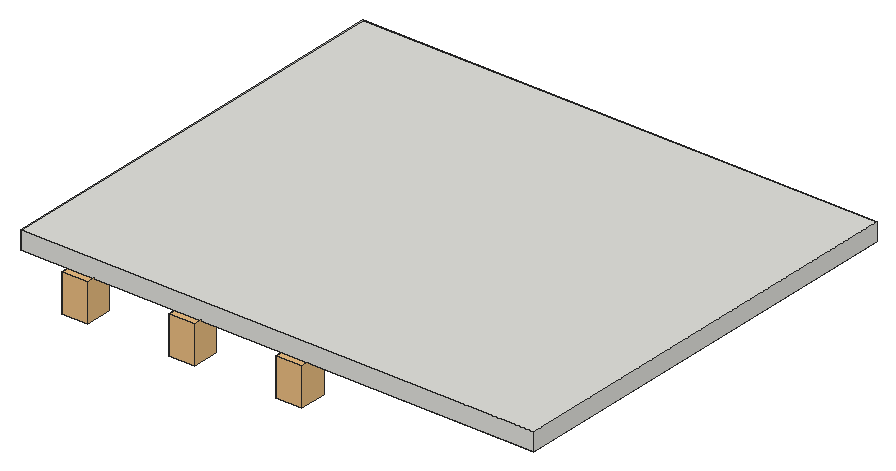
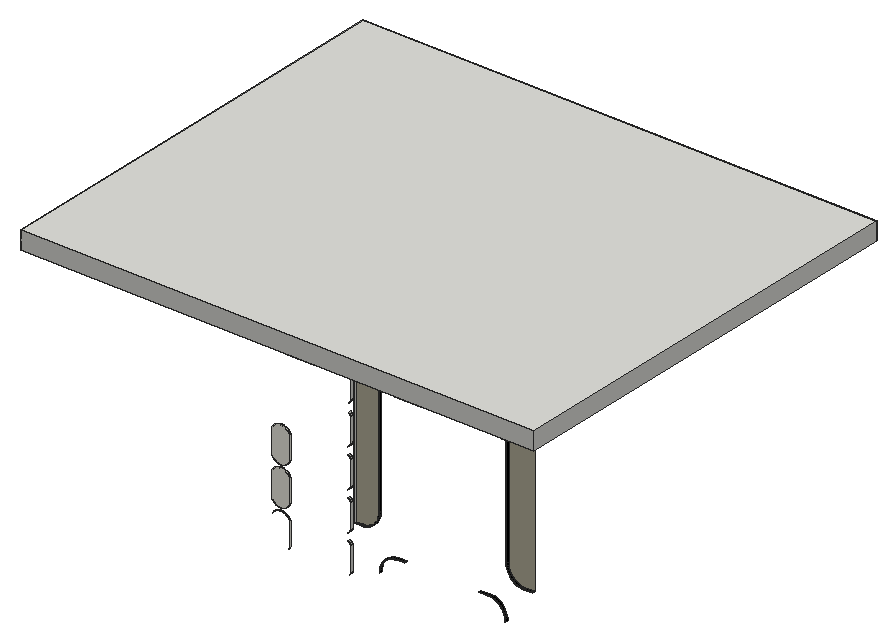
# SketchUp Ruby script. Lengths in inches.
U = 1.inch
M = Sketchup.active_model
def pt(a) = Geom::Point3d.new(a.map { |v| v * U })
def face(e, loops, mat)
  f = e.add_face(loops[0].map { |a| pt(a) })
  loops[1..].each { |l| e.add_face(l.map { |a| pt(a) }).erase! }
  f.material = f.back_material = mat if mat
  f
end
# faces: each face lists its corners as indices into pts; further lists are holes
def faces(e, pts, list, mat = nil) = list.each { |f| face(e, (f[0].is_a?(Array) ? f : [f]).map { |l| l.map { |i| pts[i] } }, mat) }
# xy, xz, yz: faces in a plane at the given z, y or x. An outline is a flat list of corners, or four numbers for a rectangle; further outlines are holes
def ring(l) = l.size == 4 ? [[l[0], l[1]], [l[2], l[1]], [l[2], l[3]], [l[0], l[3]]] : l.each_slice(2).to_a
def flat(e, list, mat, &to3) = list.each { |f| face(e, (f[0].is_a?(Array) ? f : [f]).map { |l| ring(l).map { |u, v| to3.(u, v) } }, mat) }
def xy(e, z, list, mat = nil) = flat(e, list, mat) { |x, y| [x, y, z] }
def xz(e, y, list, mat = nil) = flat(e, list, mat) { |x, z| [x, y, z] }
def yz(e, x, list, mat = nil) = flat(e, list, mat) { |y, z| [x, y, z] }
def lines(e, pts, list) = list.each { |a, b| e.add_line(pt(pts[a]), pt(pts[b])) }
# prism: a flat outline (further loops are holes) pulled along v
def prism(e, loops, v, mat = nil)
  f = face(e, loops, mat); d = Geom::Vector3d.new(v.map { |x| x * U })
  f.pushpull(f.normal.samedirection?(d) ? d.length : -d.length)
end
def box(e, o, s, mat = nil) = prism(e, [[o, [o[0] + s[0], o[1], o[2]], [o[0] + s[0], o[1] + s[1], o[2]], [o[0], o[1] + s[1], o[2]]]], [0, 0, s[2]], mat)
def at(x, y, z, deg = 0) = Geom::Transformation.translation(pt([x, y, z])) * Geom::Transformation.rotation(ORIGIN, Z_AXIS, deg.degrees)
def axes(o, x, y, z) = Geom::Transformation.new([*x, 0, *y, 0, *z, 0, *pt(o).to_a, 1])
def part(name) = M.definitions.add(name)
# library, detail: a bought-in or finely detailed component or shape, given as its bounding box
def library(name, o, s) = part(name).tap { |d| box(d.entities, o, s) }
def detail(e, o, s) = box(e.add_group.entities, o, s)
def put(e, d, t, mat = nil) = e.add_instance(d, t).tap { |i| i.material = mat if mat }
def group(e, t, mat = nil) = e.add_group.tap { |g| g.transformation = t; g.material = mat if mat }.entities
root = M.entities
M.materials.add("Tafisa-Gardenia-or-Gardenia-PM775-4K").color = [246, 245, 235]
M.materials.add("Uniboard-L19-Putty-4K").color = [187, 181, 160]
M.materials.add("[Color M09]").color = [0, 0, 0]
c1 = library("Group\#8",[0,0,0],[8.9,8.9,12.62])
xy(root,61.26,[[19.5,138,22.5,138.71],[47.5,138,50,138.71]],"[Color M09]")
xy(root,61.5,[[19.5,138,22.5,138.71],[47.5,138,50,138.71]],"[Color M09]")
xy(root,67.3125,[[4.5,138,7.5,138.71],[62,138,64.38,138.71]],"[Color M09]")
xy(root,67.55,[[4.5,138,7.5,138.71],[62,138,64.38,138.71]],"[Color M09]")
xz(root,138,[[4.5,67.55,7.5,67.55,8.25,67.6,8.99,67.75,9.71,67.99,10.38,68.32,11.01,68.74,11.58,69.24,12.07,69.8,12.49,70.43,12.83,71.11,13.07,71.82,13.21,72.56,13.26,73.3125,13.26,114,4.5,114],[62,67.55,64.38,67.55,64.38,114,56.24,114,56.24,73.3125,56.29,72.56,56.43,71.82,56.67,71.11,57.01,70.43,57.43,69.8,57.92,69.24,58.49,68.74,59.12,68.32,59.79,67.99,60.51,67.75,61.25,67.6]],"Uniboard-L19-Putty-4K")
xz(root,138.25,[[89.53,63,89.85,63.02,90.17,63.0625,90.48,63.14,90.78,63.25,91.07,63.38,91.35,63.55,91.61,63.73,91.84,63.95,92.0625,64.18,92.25,64.4375,92.42,64.71,92.5625,65,92.5625,73,92.42,73.29,92.25,73.5625,92.0625,73.82,91.84,74.05,91.61,74.27,91.35,74.45,91.07,74.62,90.78,74.75,90.48,74.86,90.17,74.9375,89.85,74.98,89.53,75,89.21,74.98,89.02,74.96,88.89,74.9375,88.58,74.86,88.28,74.75,87.99,74.62,87.72,74.45,87.46,74.27,87.22,74.05,87,73.82,86.81,73.5625,86.64,73.29,86.5,73,86.5,65,86.64,64.71,86.81,64.4375,87,64.18,87.22,63.95,87.46,63.73,87.72,63.55,87.99,63.38,88.28,63.25,88.58,63.14,88.89,63.0625,89.02,63.04,89.21,63.02],[89.53,76,89.85,76.02,90.17,76.0625,90.48,76.14,90.78,76.25,91.07,76.38,91.35,76.55,91.61,76.73,91.84,76.95,92.0625,77.18,92.25,77.4375,92.42,77.71,92.5625,78,92.5625,86,92.42,86.29,92.25,86.5625,92.0625,86.82,91.84,87.05,91.61,87.27,91.35,87.45,91.07,87.62,90.78,87.75,90.48,87.86,90.17,87.9375,89.85,87.98,89.53,88,89.21,87.98,88.89,87.9375,88.58,87.86,88.28,87.75,87.99,87.62,87.72,87.45,87.46,87.27,87.22,87.05,87,86.82,86.81,86.5625,86.64,86.29,86.5,86,86.5,78,86.64,77.71,86.81,77.4375,87,77.18,87.22,76.95,87.46,76.73,87.72,76.55,87.99,76.38,88.28,76.25,88.58,76.14,88.89,76.0625,89.02,76.04,89.21,76.02]],"Tafisa-Gardenia-or-Gardenia-PM775-4K")
yz(root,13.26,[[138,73.3125,138.71,114]],"[Color M09]")
yz(root,13.5,[[138,73.3125,138.71,114]],"[Color M09]")
yz(root,56,[[138,73.3125,138.71,114]],"[Color M09]")
yz(root,56.24,[[138,73.3125,138.71,114]],"[Color M09]")
yz(root,64.38,[[138,67.55,138.71,114]])
yz(root,64.5,[[138,67.3125,138.71,67.55],[138,67.55,138.71,114]])
yz(root,65.5,[[138,52,138.79,60],[138,65,138.79,73],[138,78,138.79,86],[138,91,138.79,99],[138,104,138.79,112]])
yz(root,86.5,[[138,52,138.25,60],[138,65,138.25,73],[138,78,138.25,86]],"Tafisa-Gardenia-or-Gardenia-PM775-4K")
p = [[65.8,138.79,51.44],[65.64,138.79,51.71],[65.64,138,51.71],[65.8,138,51.44],[86.64,138,51.71],[86.81,138,51.4375],
  [86.81,138.25,51.4375],[86.64,138.25,51.71],[65.5,138.79,52],[65.5,138,52],[86.5,138,52],[86.5,138.25,52],
  [13.55,138,56.28],[13.5,138,55.5],[13.5,138.71,55.5],[13.55,138.71,56.28],[13.74,138,55.5],[13.79,138,56.25],
  [13.79,138.71,56.25],[13.74,138.71,55.5],[55.71,138,56.25],[55.76,138,55.5],[55.76,138.71,55.5],[55.71,138.71,56.25],
  [56,138,55.5],[55.95,138,56.28],[55.95,138.71,56.28],[56,138.71,55.5],[13.7,138,57.05],[13.7,138.71,57.05],
  [13.93,138,56.99],[13.93,138.71,56.99],[55.57,138,56.99],[55.57,138.71,56.99],[55.8,138,57.05],[55.8,138.71,57.05],
  [14.17,138,57.71],[14.17,138.71,57.71],[55.33,138,57.71],[55.33,138.71,57.71],[13.96,138,57.8],[13.96,138.71,57.8],
  [55.54,138,57.8],[55.54,138.71,57.8],[14.51,138,58.38],[14.51,138.71,58.38],[54.99,138,58.38],[54.99,138.71,58.38],
  [14.3,138,58.5],[14.3,138.71,58.5],[55.2,138,58.5],[55.2,138.71,58.5],[14.93,138,59.01],[14.93,138.71,59.01],
  [54.57,138,59.01],[54.57,138.71,59.01],[14.74,138,59.15],[14.74,138.71,59.15],[54.76,138,59.15],[54.76,138.71,59.15],
  [15.42,138,59.58],[15.42,138.71,59.58],[54.08,138,59.58],[54.08,138.71,59.58],[15.26,138,59.74],[15.26,138.71,59.74],
  [54.24,138,59.74],[54.24,138.71,59.74],[15.99,138,60.07],[15.99,138.71,60.07],[53.51,138,60.07],[53.51,138.71,60.07],
  [15.85,138,60.26],[15.85,138.71,60.26],[53.65,138,60.26],[53.65,138.71,60.26],[65.5,138.79,60],[65.64,138.79,60.29],
  [65.64,138,60.29],[65.5,138,60],[86.64,138,60.29],[86.5,138,60],[86.5,138.25,60],[86.64,138.25,60.29],
  [16.62,138,60.49],[16.62,138.71,60.49],[52.88,138,60.49],[52.88,138.71,60.49],[16.5,138,60.7],[16.5,138.71,60.7],
  [53,138,60.7],[53,138.71,60.7],[65.8,138.79,60.56],[65.8,138,60.56],[86.81,138,60.5625],[86.81,138.25,60.5625],
  [17.29,138,60.83],[17.29,138.71,60.83],[52.21,138,60.83],[52.21,138.71,60.83],[65.99,138.79,60.82],[65.99,138,60.82],
  [87,138,60.82],[87,138.25,60.82],[92.25,138,60.5625],[92.0625,138,60.82],[92.0625,138.25,60.82],[92.25,138.25,60.5625],
  [17.2,138,61.04],[17.2,138.71,61.04],[52.3,138,61.04],[52.3,138.71,61.04],[18.01,138,61.07],[18.01,138.71,61.07],
  [51.49,138,61.07],[51.49,138.71,61.07],[66.21,138.79,61.05],[66.21,138,61.05],[87.22,138,61.05],[87.22,138.25,61.05],
  [91.84,138,61.05],[91.84,138.25,61.05],[17.95,138,61.3],[17.95,138.71,61.3],[51.55,138,61.3],[51.55,138.71,61.3],
  [18.75,138,61.21],[18.75,138.71,61.21],[50.75,138,61.21],[50.75,138.71,61.21],[66.44,138.79,61.26],[66.44,138,61.26],
  [87.46,138,61.27],[87.46,138.25,61.27],[91.61,138,61.27],[91.61,138.25,61.27],[19.5,138,61.26],[19.5,138.71,61.26],
  [50,138,61.26],[50,138.71,61.26],[18.72,138,61.45],[18.72,138.71,61.45],[50.78,138,61.45],[50.78,138.71,61.45],
  [87.72,138,61.45],[87.72,138.25,61.45],[91.35,138,61.45],[91.35,138.25,61.45],[19.5,138,61.5],[19.5,138.71,61.5],
  [50,138,61.5],[50,138.71,61.5],[87.99,138,61.62],[87.99,138.25,61.62],[91.07,138,61.62],[91.07,138.25,61.62],
  [88.28,138,61.75],[88.28,138.25,61.75],[90.78,138,61.75],[90.78,138.25,61.75],[88.58,138,61.86],[88.58,138.25,61.86],
  [90.48,138,61.86],[90.48,138.25,61.86],[88.89,138,61.9375],[88.89,138.25,61.9375],[89.02,138,61.96],[89.02,138.25,61.96],
  [90.17,138,61.9375],[89.85,138,61.98],[89.85,138.25,61.98],[90.17,138.25,61.9375],[89.21,138,61.98],[89.21,138.25,61.98],
  [89.53,138,62],[89.53,138.25,62],[88.89,138,63.0625],[89.02,138,63.04],[89.02,138.25,63.04],[88.89,138.25,63.0625],
  [89.21,138,63.02],[89.21,138.25,63.02],[89.53,138,63],[89.53,138.25,63],[89.85,138,63.02],[89.85,138.25,63.02],
  [90.17,138,63.0625],[90.17,138.25,63.0625],[88.28,138,63.25],[88.58,138,63.14],[88.58,138.25,63.14],[88.28,138.25,63.25],
  [88.78,138,63.09],[88.78,138.25,63.09],[90.48,138,63.14],[90.48,138.25,63.14],[90.78,138,63.25],[90.78,138.25,63.25],
  [87.99,138,63.38],[87.99,138.25,63.38],[91.07,138,63.38],[91.07,138.25,63.38],[87.72,138,63.55],[87.72,138.25,63.55],
  [91.35,138,63.55],[91.35,138.25,63.55],[87.46,138,63.73],[87.46,138.25,63.73],[91.61,138,63.73],[91.61,138.25,63.73],
  [66.44,138.79,63.74],[66.21,138.79,63.95],[66.21,138,63.95],[66.44,138,63.74],[87.22,138,63.95],[87.22,138.25,63.95],
  [91.84,138,63.95],[91.84,138.25,63.95],[65.99,138.79,64.18],[65.99,138,64.18],[87,138,64.18],[87,138.25,64.18],
  [92.0625,138,64.18],[92.0625,138.25,64.18],[65.8,138.79,64.44],[65.8,138,64.44],[86.81,138,64.4375],[86.81,138.25,64.4375],
  [92.25,138,64.4375],[92.25,138.25,64.4375],[65.64,138.79,64.71],[65.64,138,64.71],[86.64,138,64.71],[86.64,138.25,64.71],
  [65.5,138.79,65],[65.5,138,65],[86.5,138,65],[86.5,138.25,65],[7.5,138,67.3125],[8.28,138,67.36],
  [8.28,138.71,67.36],[7.5,138.71,67.3125],[61.22,138,67.36],[62,138,67.3125],[62,138.71,67.3125],[61.22,138.71,67.36],
  [9.05,138,67.52],[9.05,138.71,67.52],[60.45,138,67.52],[60.45,138.71,67.52],[8.25,138,67.6],[7.5,138,67.55],
  [7.5,138.71,67.55],[8.25,138.71,67.6],[9.8,138,67.77],[9.8,138.71,67.77],[59.7,138,67.77],[59.7,138.71,67.77],
  [62,138,67.55],[61.25,138,67.6],[61.25,138.71,67.6],[62,138.71,67.55],[8.99,138,67.75],[8.99,138.71,67.75],
  [60.51,138,67.75],[60.51,138.71,67.75],[9.71,138,67.99],[9.71,138.71,67.99],[59.79,138,67.99],[59.79,138.71,67.99],
  [10.5,138,68.12],[10.5,138.71,68.12],[59,138,68.12],[59,138.71,68.12],[10.38,138,68.32],[10.38,138.71,68.32],
  [59.12,138,68.32],[59.12,138.71,68.32],[11.15,138,68.55],[11.15,138.71,68.55],[58.35,138,68.55],[58.35,138.71,68.55],
  [11.01,138,68.74],[11.01,138.71,68.74],[58.49,138,68.74],[58.49,138.71,68.74],[11.74,138,69.07],[11.74,138.71,69.07],
  [57.76,138,69.07],[57.76,138.71,69.07],[11.58,138,69.24],[11.58,138.71,69.24],[57.92,138,69.24],[57.92,138.71,69.24],
  [12.26,138,69.66],[12.26,138.71,69.66],[57.24,138,69.66],[57.24,138.71,69.66],[12.07,138,69.8],[12.07,138.71,69.8],
  [57.43,138,69.8],[57.43,138.71,69.8],[12.7,138,70.3125],[12.7,138.71,70.3125],[56.8,138,70.3125],[56.8,138.71,70.3125],
  [12.49,138,70.43],[12.49,138.71,70.43],[57.01,138,70.43],[57.01,138.71,70.43],[13.04,138,71.02],[13.04,138.71,71.02],
  [56.46,138,71.02],[56.46,138.71,71.02],[12.83,138,71.11],[12.83,138.71,71.11],[56.67,138,71.11],[56.67,138.71,71.11],
  [13.3,138,71.76],[13.3,138.71,71.76],[56.2,138,71.76],[56.2,138.71,71.76],[13.07,138,71.82],[13.07,138.71,71.82],
  [56.43,138,71.82],[56.43,138.71,71.82],[13.21,138,72.56],[13.21,138.71,72.56],[13.45,138,72.53],[13.45,138.71,72.53],
  [56.05,138,72.53],[56.05,138.71,72.53],[56.29,138,72.56],[56.29,138.71,72.56],[13.5,138,73.3125],[13.5,138.71,73.3125],
  [56,138,73.3125],[56,138.71,73.3125],[13.26,138,73.3125],[13.26,138.71,73.3125],[56.24,138,73.3125],[56.24,138.71,73.3125],
  [65.5,138.79,73],[65.64,138.79,73.29],[65.64,138,73.29],[65.5,138,73],[86.64,138,73.29],[86.5,138,73],
  [86.5,138.25,73],[86.64,138.25,73.29],[65.8,138.79,73.56],[65.8,138,73.56],[86.81,138,73.5625],[86.81,138.25,73.5625],
  [65.99,138.79,73.82],[65.99,138,73.82],[87,138,73.82],[87,138.25,73.82],[66.21,138.79,74.05],[66.21,138,74.05],
  [87.22,138,74.05],[87.22,138.25,74.05],[92.0625,138,73.82],[91.84,138,74.05],[91.84,138.25,74.05],[92.0625,138.25,73.82],
  [66.44,138.79,74.26],[66.44,138,74.26],[87.46,138,74.27],[87.46,138.25,74.27],[91.61,138,74.27],[91.61,138.25,74.27],
  [87.72,138,74.45],[87.72,138.25,74.45],[91.35,138,74.45],[91.35,138.25,74.45],[87.99,138,74.62],[87.99,138.25,74.62],
  [91.07,138,74.62],[91.07,138.25,74.62],[88.28,138,74.75],[88.28,138.25,74.75],[90.78,138,74.75],[90.78,138.25,74.75],
  [88.58,138,74.86],[88.58,138.25,74.86],[90.48,138,74.86],[90.48,138.25,74.86],[88.89,138,74.9375],[88.89,138.25,74.9375],
  [89.02,138,74.96],[89.02,138.25,74.96],[90.17,138,74.9375],[89.85,138,74.98],[89.85,138.25,74.98],[90.17,138.25,74.9375],
  [89.21,138,74.98],[89.21,138.25,74.98],[89.53,138,75],[89.53,138.25,75],[88.89,138,76.0625],[89.02,138,76.04],
  [89.02,138.25,76.04],[88.89,138.25,76.0625],[89.21,138,76.02],[89.21,138.25,76.02],[89.53,138,76],[89.53,138.25,76],
  [89.85,138,76.02],[89.85,138.25,76.02],[90.17,138,76.0625],[90.17,138.25,76.0625],[88.28,138,76.25],[88.58,138,76.14],
  [88.58,138.25,76.14],[88.28,138.25,76.25],[90.48,138,76.14],[90.48,138.25,76.14],[90.78,138,76.25],[90.78,138.25,76.25],
  [87.99,138,76.38],[87.99,138.25,76.38],[91.07,138,76.38],[91.07,138.25,76.38],[87.72,138,76.55],[87.72,138.25,76.55],
  [91.35,138,76.55],[91.35,138.25,76.55],[87.46,138,76.73],[87.46,138.25,76.73],[91.61,138,76.73],[91.61,138.25,76.73],
  [66.44,138.79,76.74],[66.21,138.79,76.95],[66.21,138,76.95],[66.44,138,76.74],[87.22,138,76.95],[87.22,138.25,76.95],
  [91.84,138,76.95],[91.84,138.25,76.95],[65.99,138.79,77.18],[65.99,138,77.18],[87,138,77.18],[87,138.25,77.18],
  [92.0625,138,77.18],[92.0625,138.25,77.18],[65.8,138.79,77.44],[65.8,138,77.44],[86.81,138,77.4375],[86.81,138.25,77.4375],
  [65.64,138.79,77.71],[65.64,138,77.71],[86.64,138,77.71],[86.64,138.25,77.71],[65.5,138.79,78],[65.5,138,78],
  [86.5,138,78],[86.5,138.25,78],[65.5,138.79,86],[65.64,138.79,86.29],[65.64,138,86.29],[65.5,138,86],
  [86.64,138,86.29],[86.5,138,86],[86.5,138.25,86],[86.64,138.25,86.29],[65.8,138.79,86.56],[65.8,138,86.56],
  [86.81,138,86.5625],[86.81,138.25,86.5625],[65.99,138.79,86.82],[65.99,138,86.82],[87,138,86.82],[87,138.25,86.82],
  [66.21,138.79,87.05],[66.21,138,87.05],[87.22,138,87.05],[87.22,138.25,87.05],[92.0625,138,86.82],[91.84,138,87.05],
  [91.84,138.25,87.05],[92.0625,138.25,86.82],[66.44,138.79,87.26],[66.44,138,87.26],[87.46,138,87.27],[87.46,138.25,87.27],
  [91.61,138,87.27],[91.61,138.25,87.27],[87.72,138,87.45],[87.72,138.25,87.45],[91.35,138,87.45],[91.35,138.25,87.45],
  [87.99,138,87.62],[87.99,138.25,87.62],[91.07,138,87.62],[91.07,138.25,87.62],[88.28,138,87.75],[88.28,138.25,87.75],
  [90.78,138,87.75],[90.78,138.25,87.75],[88.58,138,87.86],[88.58,138.25,87.86],[90.48,138,87.86],[90.48,138.25,87.86],
  [88.89,138,87.9375],[88.89,138.25,87.9375],[89.21,138,87.98],[89.21,138.25,87.98],[90.17,138,87.9375],[89.85,138,87.98],
  [89.85,138.25,87.98],[90.17,138.25,87.9375],[89.53,138,88],[89.53,138.25,88],[66.44,138.79,89.74],[66.21,138.79,89.95],
  [66.21,138,89.95],[66.44,138,89.74],[65.99,138.79,90.18],[65.99,138,90.18],[65.8,138.79,90.44],[65.8,138,90.44],
  [65.64,138.79,90.71],[65.64,138,90.71],[65.5,138.79,91],[65.5,138,91],[65.5,138.79,99],[65.64,138.79,99.29],
  [65.64,138,99.29],[65.5,138,99],[65.8,138.79,99.56],[65.8,138,99.56],[65.99,138.79,99.82],[65.99,138,99.82],
  [66.21,138.79,100.05],[66.21,138,100.05],[66.21,138.79,102.95],[65.99,138.79,103.18],[65.99,138,103.18],[66.21,138,102.95],
  [65.8,138.79,103.44],[65.8,138,103.44],[65.64,138.79,103.71],[65.64,138,103.71],[65.5,138.79,104],[65.5,138,104],
  [65.5,138.79,112],[65.64,138.79,112.29],[65.64,138,112.29],[65.5,138,112],[65.8,138.79,112.56],[65.8,138,112.56],
  [65.99,138.79,112.82],[65.99,138,112.82],[66.21,138.79,113.05],[66.21,138,113.05]]
faces(root,p,[[0,1,2,3],[1,8,9,2],[76,77,78,79],[77,92,93,78],[92,100,101,93],[100,116,117,101],[116,130,131,117],[210,211,212,213],
  [211,218,219,212],[218,224,225,219],[224,230,231,225],[230,234,235,231],[342,343,344,345],[343,350,351,344],[350,354,355,351],[354,358,359,355],
  [358,366,367,359],[432,433,434,435],[433,440,441,434],[440,446,447,441],[446,450,451,447],[450,454,455,451],[458,459,460,461],[459,466,467,460],
  [466,470,471,467],[470,474,475,471],[474,482,483,475],[514,515,516,517],[515,518,519,516],[518,520,521,519],[520,522,523,521],[522,524,525,523],
  [526,527,528,529],[527,530,531,528],[530,532,533,531],[532,534,535,533],[536,537,538,539],[537,540,541,538],[540,542,543,541],[542,544,545,543],
  [546,547,548,549],[547,550,551,548],[550,552,553,551],[552,554,555,553]])
faces(root,p,[[4,5,6,7],[10,4,7,11],[80,81,82,83],[94,80,83,95],[102,94,95,103],[104,105,106,107],[118,102,103,119],[105,120,121,106],
  [132,118,119,133],[120,134,135,121],[144,132,133,145],[134,146,147,135],[152,144,145,153],[146,154,155,147],[156,152,153,157],[154,158,159,155],
  [160,156,157,161],[158,162,163,159],[164,160,161,165],[166,164,165,167],[168,169,170,171],[162,168,171,163],[172,166,167,173],[174,172,173,175],
  [169,174,175,170],[176,177,178,179],[177,180,181,178],[180,182,183,181],[182,184,185,183],[184,186,187,185],[188,189,190,191],[189,192,193,190],
  [192,176,179,193],[186,194,195,187],[194,196,197,195],[198,188,191,199],[196,200,201,197],[202,198,199,203],[200,204,205,201],[206,202,203,207],
  [204,208,209,205],[214,206,207,215],[208,216,217,209],[220,214,215,221],[216,222,223,217],[226,220,221,227],[222,228,229,223],[232,226,227,233],
  [236,232,233,237],[346,347,348,349],[352,346,349,353],[356,352,353,357],[360,356,357,361],[362,363,364,365],[368,360,361,369],[363,370,371,364],
  [372,368,369,373],[370,374,375,371],[376,372,373,377],[374,378,379,375],[380,376,377,381],[378,382,383,379],[384,380,381,385],[382,386,387,383],
  [388,384,385,389],[390,388,389,391],[392,393,394,395],[386,392,395,387],[396,390,391,397],[398,396,397,399],[393,398,399,394],[400,401,402,403],
  [401,404,405,402],[404,406,407,405],[406,408,409,407],[408,410,411,409],[412,413,414,415],[413,400,403,414],[410,416,417,411],[416,418,419,417],
  [420,412,415,421],[418,422,423,419],[424,420,421,425],[422,426,427,423],[428,424,425,429],[426,430,431,427],[436,428,429,437],[430,438,439,431],
  [442,436,437,443],[438,444,445,439],[448,442,443,449],[452,448,449,453],[456,452,453,457],[462,463,464,465],[468,462,465,469],[472,468,469,473],
  [476,472,473,477],[478,479,480,481],[484,476,477,485],[479,486,487,480],[488,484,485,489],[486,490,491,487],[492,488,489,493],[490,494,495,491],
  [496,492,493,497],[494,498,499,495],[500,496,497,501],[498,502,503,499],[504,500,501,505],[506,504,505,507],[508,509,510,511],[502,508,511,503],
  [512,506,507,513],[509,512,513,510]],"Tafisa-Gardenia-or-Gardenia-PM775-4K")
faces(root,p,[[12,13,14,15],[16,17,18,19],[20,21,22,23],[24,25,26,27],[28,12,15,29],[17,30,31,18],[32,20,23,33],[25,34,35,26],
  [30,36,37,31],[38,32,33,39],[40,28,29,41],[34,42,43,35],[36,44,45,37],[46,38,39,47],[48,40,41,49],[42,50,51,43],
  [44,52,53,45],[54,46,47,55],[56,48,49,57],[50,58,59,51],[52,60,61,53],[62,54,55,63],[64,56,57,65],[58,66,67,59],
  [60,68,69,61],[70,62,63,71],[72,64,65,73],[66,74,75,67],[68,84,85,69],[86,70,71,87],[88,72,73,89],[74,90,91,75],
  [84,96,97,85],[98,86,87,99],[108,88,89,109],[90,110,111,91],[96,112,113,97],[114,98,99,115],[122,108,109,123],[110,124,125,111],
  [112,126,127,113],[128,114,115,129],[126,136,137,127],[138,128,129,139],[140,122,123,141],[124,142,143,125],[148,140,141,149],[142,150,151,143],
  [238,239,240,241],[242,243,244,245],[239,246,247,240],[248,242,245,249],[250,251,252,253],[246,254,255,247],[256,248,249,257],[258,259,260,261],
  [262,250,253,263],[259,264,265,260],[266,262,263,267],[264,268,269,265],[254,270,271,255],[272,256,257,273],[274,266,267,275],[268,276,277,269],
  [270,278,279,271],[280,272,273,281],[282,274,275,283],[276,284,285,277],[278,286,287,279],[288,280,281,289],[290,282,283,291],[284,292,293,285],
  [286,294,295,287],[296,288,289,297],[298,290,291,299],[292,300,301,293],[294,302,303,295],[304,296,297,305],[306,298,299,307],[300,308,309,301],
  [302,310,311,303],[312,304,305,313],[314,306,307,315],[308,316,317,309],[310,318,319,311],[320,312,313,321],[322,314,315,323],[316,324,325,317],
  [326,322,323,327],[318,328,329,319],[330,320,321,331],[324,332,333,325],[328,334,335,329],[336,330,331,337],[338,326,327,339],[332,340,341,333]],"[Color M09]")
put(root,c1,at(15.66,-2.26,101.38))
put(root,c1,at(51.66,-2.26,101.38))
put(root,c1,at(87.66,-2.26,101.38))
put(root,c1,at(15.66,27.74,101.38))
put(root,c1,at(51.66,27.74,101.38))
put(root,c1,at(87.66,27.74,101.38))
put(root,c1,at(15.66,57.74,101.38))
put(root,c1,at(51.66,57.74,101.38))
put(root,c1,at(87.66,57.74,101.38))
g1 = group(root,at(0,0,114))
box(g1,[0,0,0],[172.5,144,6])
put(root,c1,at(15.66,87.74,101.38))
put(root,c1,at(51.66,87.74,101.38))
put(root,c1,at(87.66,87.74,101.38))
put(root,c1,at(15.66,117.74,101.38))
put(root,c1,at(51.66,117.74,101.38))
put(root,c1,at(87.66,117.74,101.38))
